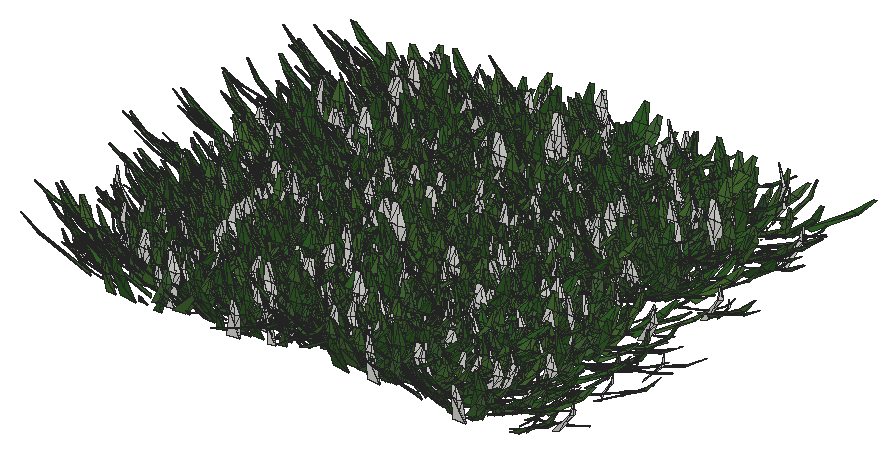
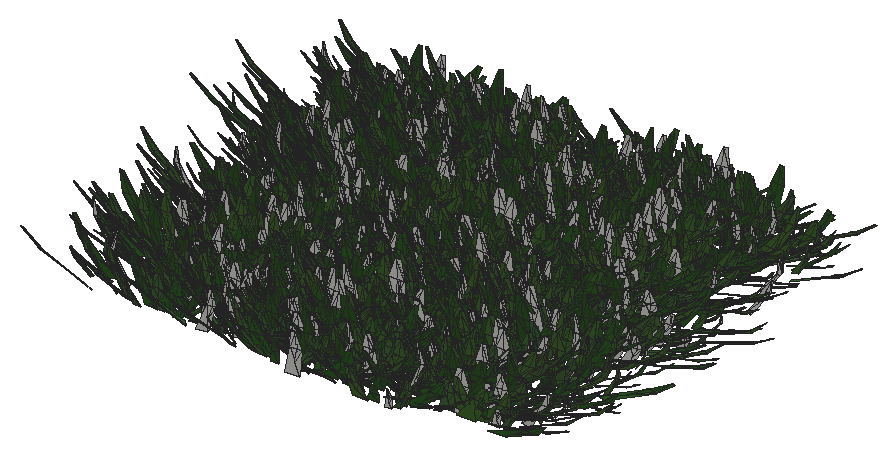
# SketchUp Ruby script. Lengths in inches.
U = 1.inch
M = Sketchup.active_model
def pt(a) = Geom::Point3d.new(a.map { |v| v * U })
def face(e, loops, mat)
  f = e.add_face(loops[0].map { |a| pt(a) })
  loops[1..].each { |l| e.add_face(l.map { |a| pt(a) }).erase! }
  f.material = f.back_material = mat if mat
  f
end
# faces: each face lists its corners as indices into pts; further lists are holes
def faces(e, pts, list, mat = nil) = list.each { |f| face(e, (f[0].is_a?(Array) ? f : [f]).map { |l| l.map { |i| pts[i] } }, mat) }
# xy, xz, yz: faces in a plane at the given z, y or x. An outline is a flat list of corners, or four numbers for a rectangle; further outlines are holes
def ring(l) = l.size == 4 ? [[l[0], l[1]], [l[2], l[1]], [l[2], l[3]], [l[0], l[3]]] : l.each_slice(2).to_a
def flat(e, list, mat, &to3) = list.each { |f| face(e, (f[0].is_a?(Array) ? f : [f]).map { |l| ring(l).map { |u, v| to3.(u, v) } }, mat) }
def xy(e, z, list, mat = nil) = flat(e, list, mat) { |x, y| [x, y, z] }
def xz(e, y, list, mat = nil) = flat(e, list, mat) { |x, z| [x, y, z] }
def yz(e, x, list, mat = nil) = flat(e, list, mat) { |y, z| [x, y, z] }
def lines(e, pts, list) = list.each { |a, b| e.add_line(pt(pts[a]), pt(pts[b])) }
# prism: a flat outline (further loops are holes) pulled along v
def prism(e, loops, v, mat = nil)
  f = face(e, loops, mat); d = Geom::Vector3d.new(v.map { |x| x * U })
  f.pushpull(f.normal.samedirection?(d) ? d.length : -d.length)
end
def box(e, o, s, mat = nil) = prism(e, [[o, [o[0] + s[0], o[1], o[2]], [o[0] + s[0], o[1] + s[1], o[2]], [o[0], o[1] + s[1], o[2]]]], [0, 0, s[2]], mat)
def at(x, y, z, deg = 0) = Geom::Transformation.translation(pt([x, y, z])) * Geom::Transformation.rotation(ORIGIN, Z_AXIS, deg.degrees)
def axes(o, x, y, z) = Geom::Transformation.new([*x, 0, *y, 0, *z, 0, *pt(o).to_a, 1])
def part(name) = M.definitions.add(name)
# library, detail: a bought-in or finely detailed component or shape, given as its bounding box
def library(name, o, s) = part(name).tap { |d| box(d.entities, o, s) }
def detail(e, o, s) = box(e.add_group.entities, o, s)
def put(e, d, t, mat = nil) = e.add_instance(d, t).tap { |i| i.material = mat if mat }
def group(e, t, mat = nil) = e.add_group.tap { |g| g.transformation = t; g.material = mat if mat }.entities
root = M.entities
M.materials.add("Material10").color = [48, 100, 38]
M.materials.add("Material3").color = [68, 110, 58]
M.materials.add("Material4").color = [48, 90, 38]
M.materials.add("Material5").color = [68, 110, 48]
M.materials.add("Material6").color = [48, 90, 48]
M.materials.add("Material7").color = [58, 110, 58]
M.materials.add("Material8").color = [58, 90, 38]
M.materials.add("Material9").color = [68, 100, 58]
c1 = part("grass00")
p = [[-0.6875,0.15,0],[-0.56,0.08,5.52],[-0.04,0.03,2.76],[0.48,-0.02,0],[0.35,-0.02,5.52],[-0.1,-0.14,5.52],
  [-0.12,0.65,8.37],[-0.42,0.65,8.37]]
faces(c1.entities,p,[[0,1,2,3],[3,2,4],[1,5,2],[5,4,2],[1,6,5],[4,5,6],[7,6,1]])
c2 = part("Group16\#1")
put(c2.entities,c1,axes([1.44,-0.61,-0.01],[0.05352,0.12609,0],[-0.10704,0.04543,0.07239],[0.06664,-0.02828,0.11628]),"Material6")
put(c2.entities,c1,axes([0.76,-0.15,-0.01],[0.04676,0.24062,0],[-0.23162,0.04501,0.06642],[0.0652,-0.01267,0.23595]),"Material3")
put(c2.entities,c1,axes([0.79,0.01,-0.01],[-0.00606,0.34651,0],[-0.34381,-0.00602,0.0432],[0.04319,0.00076,0.34386]))
put(c2.entities,c1,axes([1,0.23,-0.01],[-0.07192,0.31144,0],[-0.28722,-0.06632,0.1236],[0.12043,0.02781,0.29478]),"Material5")
put(c2.entities,c1,axes([1.66,0.77,-0.01],[-0.13828,0.29651,0],[-0.21551,-0.1005,0.22471],[0.20365,0.09498,0.23779]),"Material10")
put(c2.entities,c1,axes([0.6875,0.52,-0.01],[-0.18126,0.24051,0],[-0.22746,-0.17142,0.09788],[0.07817,0.05891,0.28481]),"Material5")
put(c2.entities,c1,axes([0.68,0.78,-0.01],[-0.215,0.18688,0],[-0.12385,-0.14248,0.21334],[0.13995,0.16101,0.18878]),"Material3")
put(c2.entities,c1,axes([0.56,1,-0.01],[-0.13756,0.07624,0],[-0.06159,-0.11112,0.0927],[0.04494,0.08108,0.12705]),"Material5")
put(c2.entities,c1,axes([0.2,0.64,-0.01],[-0.23729,0.07254,0],[-0.05711,-0.18681,0.153],[0.04473,0.14632,0.19535]),"Material10")
put(c2.entities,c1,axes([0.0625,0.72,-0.01],[-0.28874,0.02525,0],[-0.02179,-0.24916,0.14647],[0.01276,0.14591,0.25012]),"Material3")
put(c2.entities,c1,axes([-0.08,0.62,-0.01],[-0.34089,-0.04187,0],[0.03255,-0.26504,0.216],[-0.02633,0.21439,0.26703]),"Material10")
put(c2.entities,c1,axes([-0.34,0.98,-0.01],[-0.14314,-0.0493,0],[0.04397,-0.12769,0.06843],[-0.02228,0.0647,0.13505]),"Material10")
put(c2.entities,c1,axes([-0.87,1.45,-0.01],[-0.23488,-0.14114,0],[0.13761,-0.22901,0.06087],[-0.03135,0.05217,0.26717]))
put(c2.entities,c1,axes([-0.72,0.77,-0.01],[-0.14208,-0.13251,0],[0.07209,-0.0773,0.16301],[-0.11118,0.11922,0.1057]),"Material10")
put(c2.entities,c1,axes([-0.62,0.43,-0.01],[-0.14845,-0.21203,0],[0.18654,-0.13061,0.12304],[-0.10079,0.07057,0.22772]),"Material3")
put(c2.entities,c1,axes([-0.68,0.29,-0.01],[-0.13639,-0.32136,0],[0.31723,-0.13464,0.05579],[-0.05136,0.0218,0.34462]),"Material4")
put(c2.entities,c1,axes([-0.64,0.125,-0.01],[-0.0458,-0.23569,0],[0.22124,-0.043,0.08276],[-0.08124,0.01579,0.22538]),"Material7")
put(c2.entities,c1,axes([-1.6,-0.03,-0.01],[0.00576,-0.32897,0],[0.27526,0.00482,0.18018],[-0.18015,-0.00315,0.2753]),"Material5")
put(c2.entities,c1,axes([-1.36,-0.31,-0.01],[0.05718,-0.24765,0],[0.18172,0.04196,0.17267],[-0.16825,-0.03885,0.1865]),"Material10")
put(c2.entities,c1,axes([-1.54,-0.72,-0.01],[0.06537,-0.14017,0],[0.13555,0.06321,0.03939],[-0.0357,-0.01665,0.14956]))
put(c2.entities,c1,axes([-1.19,-0.9,-0.01],[0.09597,-0.12735,0],[0.11214,0.08451,0.07557],[-0.06035,-0.04548,0.14042]),"Material9")
put(c2.entities,c1,axes([-0.47,-0.54,-0.01],[0.11588,-0.10072,0],[0.0618,0.0711,0.12124],[-0.07953,-0.0915,0.0942]))
put(c2.entities,c1,axes([-0.47,-0.84,-0.01],[0.11927,-0.0661,0],[0.06603,0.11913,0.00646],[-0.00313,-0.00565,0.13621]),"Material5")
put(c2.entities,c1,axes([-0.38,-1.24,-0.01],[0.28037,-0.08571,0],[0.0618,0.20215,0.20315],[-0.05939,-0.19428,0.21139]),"Material9")
put(c2.entities,c1,axes([-0.06,-0.66,-0.01],[0.22719,-0.01987,0],[0.01247,0.14255,0.17758],[-0.01547,-0.17691,0.1431]),"Material8")
put(c2.entities,c1,axes([0.11,-0.89,-0.01],[0.14882,0.01828,0],[-0.01058,0.08611,0.12229],[0.01491,-0.12138,0.08676]),"Material6")
put(c2.entities,c1,axes([0.25,-0.72,-0.01],[0.20481,0.07053,0],[-0.06206,0.18022,0.10291],[0.03351,-0.0973,0.1906]),"Material6")
put(c2.entities,c1,axes([0.85,-1.42,-0.01],[0.16481,0.09904,0],[-0.09472,0.15762,0.05616],[0.02893,-0.04814,0.18389]),"Material5")
put(c2.entities,c1,axes([1.01,-1.09,-0.01],[0.21858,0.20385,0],[-0.17495,0.1876,0.15339],[0.10462,-0.11218,0.25652]),"Material10")
put(c2.entities,c1,axes([1.01,-0.71,-0.01],[0.08733,0.12473,0],[-0.06445,0.04512,0.13037],[0.1068,-0.07477,0.07867]),"Material6")
c3 = part("Group15\#1")
put(c3.entities,c2,at(0,0,0))
c4 = part("3darcstudiotree_grass00\#1")
put(c4.entities,c3,at(0,0,0))
put(root,c4,axes([1027.47,924.77,0],[-4.47721,-0.33604,0],[1.36403,-1.13585,-0.01736],[0.02251,-0.01875,1.33702]))
put(root,c4,axes([1027.28,911.91,0],[1.8365,-1.07849,0],[4.69569,0.49975,-0.03539],[0.15489,0.01648,1.51703]))
put(root,c4,axes([1027.77,922.46,0],[-2.97525,-0.81655,0],[2.97657,-0.67786,-0.02128],[0.12207,-0.0278,1.95268]))
put(root,c4,axes([1028.04,897.93,0],[-3.29866,-0.81098,0],[2.55083,-0.64847,-0.00764],[0.04274,-0.01087,1.81511]))
put(root,c4,axes([1028.09,930.41,0],[0.28036,-1.11473,0],[4.12363,0.06482,-0.00515],[0.03488,0.00055,1.75106]))
put(root,c4,axes([1027,915.5,0],[-2.06266,0.86143,0],[-3.87268,-0.57956,-0.03562],[-0.14938,-0.02236,1.37892]))
put(root,c4,axes([1027.79,895.99,0],[0.38604,-0.97045,0],[3.84574,0.09561,-0.03727],[0.26595,0.00661,1.73202]))
put(root,c4,axes([1028.09,899.97,0],[-3.76521,0.1423,0],[-0.75972,-1.25635,-0.03474],[-0.02334,-0.0386,1.42794]))
put(root,c4,axes([1027.06,906.23,0],[-0.0845,1.11929,0],[-4.4686,-0.02108,-0.05443],[-0.30573,-0.00144,1.56933]))
put(root,c4,axes([1028.75,921.18,0],[1.4049,-0.85059,0],[4.43609,0.45793,-0.04448],[0.26457,0.02731,1.93016]))
put(root,c4,axes([1029.04,927.01,0],[-0.32645,-1.07416,0],[4.58767,-0.08714,-0.05563],[0.36288,-0.00689,1.88098]))
put(root,c4,axes([1028.87,919.27,0],[-0.59232,1.12492,0],[-3.6265,-0.11934,-0.03263],[-0.21174,-0.00697,1.49628]))
put(root,c4,axes([1029.08,918.2,0],[4.0581,-0.29722,0],[1.26127,1.0763,-0.01036],[0.0201,0.01715,1.93559]))
put(root,c4,axes([1029.625,894.12,0],[3.20529,-0.95815,0],[3.41522,0.71406,-0.02296],[0.11616,0.02429,1.8355]))
put(root,c4,axes([1029.4,931.6,0],[-1.06603,0.92748,0],[-4.93521,-0.35453,-0.06106],[-0.26936,-0.01935,1.47293]))
put(root,c4,axes([1029.21,910.23,0],[5.08676,-0.19422,0],[0.58185,0.95246,-0.02943],[0.02798,0.0458,1.51666]))
put(root,c4,axes([1030.8,908.57,0],[-0.19939,-1.04542,0],[4.4829,-0.05344,-0.05646],[0.31576,-0.00376,1.57058]))
put(root,c4,axes([1029.35,901.36,0],[2.71383,0.81638,0],[-3.43896,0.71449,-0.05468],[-0.2392,0.0497,1.58958]))
put(root,c4,axes([1029.31,916.84,0],[4.84098,0.43489,0],[-1.61189,1.12141,-0.03831],[-0.06664,0.04636,1.53223]))
put(root,c4,axes([1029.89,928.53,0],[4.94595,-0.11829,0],[0.37031,0.96768,-0.00501],[0.00319,0.00833,1.62495]))
put(root,c4,axes([1029.56,902.87,0],[2.55592,1.10469,0],[-4.04438,0.58485,-0.02506],[-0.13578,0.01964,1.82822]))
put(root,c4,axes([1030.2,897.16,0],[4.08301,-0.07651,0],[0.38191,1.27383,-0.00347],[0.00157,0.00523,1.92949]))
put(root,c4,axes([1031.29,925.83,0],[-2.35704,0.79519,0],[-3.72282,-0.68968,-0.05517],[-0.2648,-0.04906,1.72999]))
put(root,c4,axes([1030.53,907.58,0],[2.61917,0.95948,0],[-3.03892,0.51848,-0.01403],[-0.09978,0.01702,1.97952]))
put(root,c4,axes([1030.63,913.6,0],[3.34714,0.66833,0],[-2.79001,0.87331,-0.04015],[-0.12528,0.03922,1.39698]))
put(root,c4,axes([1031.24,904.6,0],[0.48467,1.00987,0],[-3.72895,0.11185,-0.01784],[-0.13598,0.00408,1.80168]))
put(root,c4,axes([1033.03,923.72,0],[-1.59666,-0.99905,0],[3.40836,-0.34045,-0.01431],[0.10062,-0.01005,1.73701]))
put(root,c4,axes([1033.2,895.67,0],[-3.03643,0.87412,0],[-2.8621,-0.62138,-0.01448],[-0.06458,-0.01402,1.39954]))
put(root,c4,axes([1034.26,896.73,0],[-4.02149,-0.43578,0],[1.45299,-0.83803,-0.04544],[0.11799,-0.06805,1.4908]))
put(root,c4,axes([1034.54,919.36,0],[-4.89707,0.28407,0],[-0.88262,-0.95096,-0.03599],[-0.04789,-0.0516,1.43677]))
put(root,c4,axes([1033.86,904.3,0],[-3.37258,0.90608,0],[-3.64602,-0.8482,-0.01383],[-0.04832,-0.01124,1.48532]))
put(root,c4,axes([1033.36,912.23,0],[4.28972,0.40809,0],[-1.53876,1.01093,-0.01203],[-0.02546,0.01673,1.60927]))
put(root,c4,axes([1035.4,908.85,0],[-1.14965,-0.87516,0],[3.85465,-0.31648,-0.02104],[0.11481,-0.00943,1.45661]))
put(root,c4,axes([1034.59,906.46,0],[3.45148,-0.64536,0],[2.96079,0.98967,-0.02614],[0.07518,0.02513,1.48366]))
put(root,c4,axes([1035.44,910.79,0],[-4.9983,0.12378,0],[-0.36429,-0.91937,-0.0174],[-0.01281,-0.03234,1.72585]))
put(root,c4,axes([1035.97,928.63,0],[-3.38152,-0.37053,0],[1.95757,-1.11657,-0.00176],[0.00453,-0.00258,1.95594]))
put(root,c4,axes([1034.94,901.15,0],[-2.34957,0.94392,0],[-4.17021,-0.64877,-0.04897],[-0.26523,-0.04126,1.9584]))
put(root,c4,axes([1034.35,898.87,0],[3.32402,0.3596,0],[-1.44399,0.83424,-0.02703],[-0.09074,0.05242,1.9211]))
put(root,c4,axes([1036.37,916.36,0],[-3.05623,-0.47682,0],[2.41216,-0.96631,-0.00523],[0.01811,-0.00725,1.86317]))
put(root,c4,axes([1036.51,918.73,0],[-3.75382,-0.50938,0],[2.09214,-0.9636,-0.04387],[0.13012,-0.05993,1.70431]))
put(root,c4,axes([1035.75,899.8,0],[-3.73599,0.53776,0],[-2.5701,-1.11595,-0.0199],[-0.05158,-0.02239,1.67187]))
put(root,c4,axes([1034.67,915.52,0],[1.67846,0.81167,0],[-4.27264,0.55222,-0.03477],[-0.1745,0.02255,1.69826]))
put(root,c4,axes([1036.07,907.16,0],[-3.09646,0.77516,0],[-3.18498,-0.79517,-0.05526],[-0.23608,-0.05894,1.69871]))
put(root,c4,axes([1036.09,902.59,0],[2.62671,-0.96021,0],[3.1714,0.54222,-0.02882],[0.14083,0.02408,1.42183]))
put(root,c4,axes([1036.55,933.42,0],[0.41254,-1.11538,0],[3.92373,0.0907,-0.04487],[0.25663,0.00593,1.41449]))
put(root,c4,axes([1037,932.375,0],[-4.83141,-0.06367,0],[0.25709,-1.21932,-0.0488],[0.01394,-0.06614,1.65721]))
put(root,c4,axes([1036.85,894.42,0],[-3.80323,0.13534,0],[-0.55678,-0.97788,-0.03826],[-0.03613,-0.06345,1.65468]))
put(root,c4,axes([1037.46,929.85,0],[-4.67907,-0.20575,0],[0.86048,-1.22305,-0.04722],[0.03699,-0.05257,1.40384]))
put(root,c4,axes([1035.99,926.74,0],[-1.05875,1.15742,0],[-4.29725,-0.24568,-0.0233],[-0.13048,-0.00746,1.58282]))
put(root,c4,axes([1036.05,913.77,0],[4.14871,0.66652,0],[-2.80307,1.09047,-0.03131],[-0.07779,0.03026,1.48921]))
put(root,c4,axes([1036.3125,922.79,0],[2.97201,1.00736,0],[-3.97981,0.73385,-0.05484],[-0.18767,0.03461,1.31443]))
put(root,c4,axes([1036.93,921.4,0],[3.73635,0.02915,0],[-0.121,0.9694,-0.01718],[-0.00416,0.0333,1.88076]))
put(root,c4,axes([1039.2,906.45,0],[-3.38708,-0.63927,0],[2.81669,-0.93274,-0.01411],[0.04933,-0.01634,1.69584]))
put(root,c4,axes([1037.17,925.41,0],[0.16986,1.07544,0],[-5.18803,0.05121,-0.04149],[-0.19714,0.00195,1.54325]))
put(root,c4,axes([1039.4,919.5,0],[0.73918,-1.25402,0],[4.5803,0.16874,-0.00777],[0.03593,0.00132,1.3523]))
put(root,c4,axes([1039.57,916.7,0],[-0.83171,-0.90909,0],[4.59832,-0.26293,-0.04627],[0.28513,-0.0163,1.86363]))
put(root,c4,axes([1039.62,907.2,0],[-4.52783,0.09424,0],[-0.31079,-0.93327,-0.02559],[-0.01771,-0.05318,1.95328]))
put(root,c4,axes([1040.47,915.05,0],[1.09611,-0.92163,0],[4.84666,0.36027,-0.06029],[0.32691,0.0243,1.78762]))
put(root,c4,axes([1040.14,929.75,0],[2.30561,-0.85947,0],[4.07199,0.68272,-0.05795],[0.30529,0.05118,1.94389]))
put(root,c4,axes([1039.42,898.43,0],[4.15645,0.11327,0],[-0.40548,0.92998,-0.03498],[-0.02406,0.05518,1.48455]))
put(root,c4,axes([1040.35,911.98,0],[-3.28835,0.69112,0],[-2.3207,-0.69011,-0.00081],[-0.00409,-0.00122,1.76997]))
put(root,c4,axes([1041.58,924.61,0],[-0.05217,-0.99103,0],[4.9332,-0.01623,-0.00745],[0.04692,-0.00015,1.94284]))
put(root,c4,axes([1040.15,895.47,0],[0.29849,1.1081,0],[-3.91006,0.06583,-0.04154],[-0.31526,0.00531,1.86323]))
put(root,c4,axes([1041.73,921.3,0],[-4.94093,-0.24625,0],[0.95755,-1.20083,-0.01918],[0.02332,-0.02924,1.90358]))
put(root,c4,axes([1040.38,926.125,0],[3.27459,-0.53526,0],[2.01,0.76855,-0.045],[0.14728,0.05631,1.37282]))
put(root,c4,axes([1041.78,910.82,0],[0.57888,-1.02767,0],[4.86352,0.17122,-0.00524],[0.03332,0.00117,1.97007]))
put(root,c4,axes([1039.92,903.49,0],[1.77436,0.79751,0],[-3.18659,0.44311,-0.00131],[-0.00977,0.00136,1.9458]))
put(root,c4,axes([1041.04,896.86,0],[-3.36301,0.64766,0],[-2.44825,-0.79454,-0.00087],[-0.00355,-0.00115,1.68429]))
put(root,c4,axes([1042.18,901.27,0],[-1.4545,-0.88118,0],[4.51048,-0.46532,-0.01762],[0.07914,-0.00816,1.48208]))
put(root,c4,axes([1040.09,899.62,0],[3.81768,0.66428,0],[-2.44879,0.87959,-0.01513],[-0.0462,0.0166,1.43215]))
put(root,c4,axes([1041.28,922.59,0],[4.08726,-0.46656,0],[1.95644,1.0712,-0.05401],[0.10986,0.06015,1.44188]))
put(root,c4,axes([1043.09,931.68,0],[-3.9964,-0.52288,0],[2.12612,-1.01563,-0.05348],[0.15903,-0.07597,1.83786]))
put(root,c4,axes([1041.66,913.75,0],[4.81145,-0.0979,0],[0.38638,1.1868,-0.02372],[0.00959,0.02946,1.48337]))
put(root,c4,axes([1043.29,932.78,0],[-4.62401,0.29061,0],[-0.94259,-0.93738,-0.03206],[-0.05298,-0.05269,1.63785]))
put(root,c4,axes([1042.22,927.08,0],[2.68838,0.69195,0],[-3.43987,0.83529,-0.03466],[-0.15751,0.03825,1.89896]))
put(root,c4,axes([1042.27,917.97,0],[3.81617,0.61886,0],[-2.68846,1.03615,-0.05832],[-0.15316,0.05903,1.48992]))
put(root,c4,axes([1042.85,928.94,0],[-0.04272,0.99569,0],[-4.10213,-0.011,-0.03184],[-0.21296,-0.00057,1.71482]))
put(root,c4,axes([1043.27,909.27,0],[-2.13592,1.02189,0],[-4.55643,-0.59523,-0.06253],[-0.32722,-0.04275,1.89715]))
put(root,c4,axes([1043.16,904.68,0],[3.87992,-0.06992,0],[0.26674,0.92505,-0.00836],[0.00512,0.01775,1.97523]))
put(root,c4,axes([1045.57,916.74,0],[-3.92726,-0.53289,0],[2.331,-1.07368,-0.04044],[0.11775,-0.05424,1.86421]))
put(root,c4,axes([1045.87,913.58,0],[-4.06696,-0.33259,0],[1.16201,-0.88807,-0.035],[0.08068,-0.06166,1.73222]))
put(root,c4,axes([1046.48,927.5625,0],[-4.12513,-0.57559,0],[2.48785,-1.11437,-0.0179],[0.04452,-0.01994,1.62858]))
put(root,c4,axes([1045.56,901.41,0],[-3.59802,0.5872,0],[-2.6694,-1.02229,-0.04574],[-0.15156,-0.05804,1.85022]))
put(root,c4,axes([1046.375,900.48,0],[0.47235,-1.15777,0],[4.32597,0.11031,-0.00761],[0.05408,0.00138,1.94156]))
put(root,c4,axes([1046.66,919.28,0],[-3.32765,-0.85792,0],[3.0305,-0.73466,-0.04714],[0.2036,-0.04936,1.58733]))
put(root,c4,axes([1045.11,897.97,0],[5.16492,-0.13655,0],[0.53557,1.26611,-0.02611],[0.01692,0.04001,1.96192]))
put(root,c4,axes([1046.31,921.05,0],[-3.3634,0.85391,0],[-3.17768,-0.78227,-0.02428],[-0.08249,-0.02031,1.32917]))
put(root,c4,axes([1047.3,903.51,0],[-3.44,-0.36745,0],[1.97613,-1.15625,-0.04539],[0.10919,-0.06389,1.92461]))
put(root,c4,axes([1045.9,933.73,0],[4.78852,-0.11236,0],[0.42706,1.13749,-0.03728],[0.02321,0.06182,1.90298]))
put(root,c4,axes([1046.29,929.87,0],[4.63211,-0.48455,0],[1.59506,0.95302,-0.04818],[0.10631,0.06352,1.47658]))
put(root,c4,axes([1046.57,929.2,0],[3.86267,-0.07613,0],[0.40494,1.28409,-0.03935],[0.01388,0.04402,1.44542]))
put(root,c4,axes([1047.37,923.84,0],[2.43686,-0.68298,0],[3.57771,0.79783,-0.04874],[0.17486,0.03899,1.44038]))
put(root,c4,axes([1046.5,906.1,0],[4.82681,-0.00126,0],[0.00513,1.22505,-0.04894],[0.00024,0.05639,1.41164]))
put(root,c4,axes([1048.57,918.72,0],[-3.42276,-0.65167,0],[2.58269,-0.84782,-0.01582],[0.04944,-0.01623,1.37394]))
put(root,c4,axes([1047.43,915.64,0],[-2.36541,1.04526,0],[-3.84689,-0.54409,-0.02589],[-0.11432,-0.01617,1.40149]))
put(root,c4,axes([1047.96,931.86,0],[2.7424,-0.7825,0],[2.89337,0.63377,-0.00209],[0.01007,0.00221,1.54397]))
put(root,c4,axes([1048.125,926.05,0],[-4.1603,0.72793,0],[-2.33598,-0.83442,-0.01309],[-0.05536,-0.01977,1.87779]))
put(root,c4,axes([1048.86,905.07,0],[-0.84808,-1.10481,0],[3.74786,-0.17981,-0.00431],[0.02392,-0.00115,1.34772]))
put(root,c4,axes([1049.17,895.875,0],[-1.71072,-0.80836,0],[3.80701,-0.50355,-0.0302],[0.16613,-0.02197,1.67548]))
put(root,c4,axes([1049.26,908.88,0],[0.18531,-0.97415,0],[3.90679,0.04645,-0.0123],[0.08869,0.00105,1.7643]))
put(root,c4,axes([1047.97,911.875,0],[3.52409,0.23962,0],[-1.16841,1.07399,-0.02379],[-0.03363,0.03091,1.49895]))
put(root,c4,axes([1047.71,907.51,0],[1.29524,0.85298,0],[-4.77119,0.45281,-0.02635],[-0.13125,0.01246,1.69955]))
put(root,c4,axes([1049.53,922.7,0],[-4.98991,0.20865,0],[-0.7989,-1.19409,-0.00717],[-0.00589,-0.0088,1.50735]))
put(root,c4,axes([1048.97,910.96,0],[2.92176,-0.52894,0],[2.46205,0.84999,-0.04376],[0.17079,0.05896,1.7457]))
put(root,c4,axes([1051.27,916.21,0],[-2.67053,-0.99485,0],[3.36476,-0.56452,-0.00883],[0.05512,-0.00925,1.90461]))
put(root,c4,axes([1051.68,929,0],[-2.95255,-0.81537,0],[3.60487,-0.81585,-0.01753],[0.06331,-0.01433,1.48083]))
put(root,c4,axes([1049.44,896.98,0],[-0.18508,1.23432,0],[-4.73712,-0.04439,-0.00219],[-0.0103,-0.0001,1.39308]))
put(root,c4,axes([1051.89,899.52,0],[-4.20317,-0.73758,0],[2.25744,-0.80401,-0.02484],[0.09654,-0.03438,1.66133]))
put(root,c4,axes([1051.55,924.73,0],[-4.46812,0.07741,0],[-0.25002,-0.9019,-0.01842],[-0.00759,-0.0274,1.34789]))
put(root,c4,axes([1052.08,895.75,0],[-3.42874,0.45159,0],[-1.78492,-0.84701,-0.01732],[-0.06439,-0.03056,1.90951]))
put(root,c4,axes([1053.4,932.08,0],[-1.47134,-1.07173,0],[4.62951,-0.39723,-0.00214],[0.01137,-0.00098,1.72072]))
put(root,c4,axes([1051.28,900.98,0],[4.20048,0.55778,0],[-1.88075,0.88521,-0.04207],[-0.14917,0.07021,1.89419]))
put(root,c4,axes([1051.74,912.16,0],[2.35176,0.86373,0],[-3.11236,0.52965,-0.02533],[-0.14132,0.02405,1.58831]))
put(root,c4,axes([1052.4,927.66,0],[4.3887,-0.53019,0],[1.93978,1.00355,-0.00312],[0.00847,0.00438,1.73901]))
put(root,c4,axes([1052.07,907.65,0],[1.01063,1.23996,0],[-4.41491,0.2249,-0.0503],[-0.27557,0.01404,1.57458]))
put(root,c4,axes([1052.4375,918.11,0],[-1.65132,1.02753,0],[-4.1479,-0.41662,-0.02547],[-0.11726,-0.01178,1.38631]))
put(root,c4,axes([1053.59,905.59,0],[0.96836,-1.19447,0],[4.79826,0.24312,-0.041],[0.23189,0.01175,1.76588]))
put(root,c4,axes([1052.3,902.74,0],[4.53801,0.33747,0],[-1.32832,1.11639,-0.03162],[-0.04162,0.03498,1.3441]))
put(root,c4,axes([1052.14,913.24,0],[2.33175,0.74132,0],[-3.89169,0.76506,-0.01217],[-0.05632,0.01107,1.82194]))
put(root,c4,axes([1053.86,896.51,0],[1.73115,-0.99463,0],[4.00302,0.43545,-0.04597],[0.21468,0.02335,1.38947]))
put(root,c4,axes([1054.84,898.8125,0],[-4.68105,-0.44507,0],[1.39415,-0.91644,-0.04106],[0.1024,-0.06731,1.71966]))
put(root,c4,axes([1054.75,929.99,0],[-4.10991,0.05659,0],[-0.25803,-1.17127,-0.02509],[-0.00633,-0.02875,1.34616]))
put(root,c4,axes([1055.46,923.29,0],[-0.81845,-1.22057,0],[4.38476,-0.18376,-0.02808],[0.16711,-0.007,1.67665]))
put(root,c4,axes([1054.63,910.26,0],[2.60124,-1.09423,0],[3.31981,0.49325,-0.0411],[0.22316,0.03316,1.52451]))
put(root,c4,axes([1053.76,919.62,0],[3.5289,0.32153,0],[-1.76569,1.21119,-0.03532],[-0.06738,0.04622,1.79519]))
put(root,c4,axes([1054.29,915.71,0],[0.58187,0.98724,0],[-3.75225,0.13822,-0.04131],[-0.23221,0.00855,1.34689]))
put(root,c4,axes([1054.82,909.6,0],[4.31659,-0.72181,0],[2.02591,0.75722,-0.03191],[0.13976,0.05224,1.79443]))
put(root,c4,axes([1055.25,904.55,0],[3.90895,-0.31621,0],[1.44431,1.11591,-0.01717],[0.02682,0.02072,1.48777]))
put(root,c4,axes([1055.33,920.79,0],[0.60806,1.1895,0],[-3.81317,0.12183,-0.04145],[-0.33743,0.01078,1.97198]))
put(root,c4,axes([1055.06,925.64,0],[4.01339,0.62208,0],[-2.19682,0.88582,-0.03504],[-0.13521,0.05452,1.90819]))
put(root,c4,axes([1057.48,899.92,0],[-1.20844,-0.99932,0],[4.83991,-0.36579,-0.03772],[0.15637,-0.01182,1.36861]))
put(root,c4,axes([1057.26,920.68,0],[-2.41677,0.79192,0],[-3.38406,-0.64546,-0.05103],[-0.26235,-0.05004,1.72023]))
put(root,c4,axes([1057.77,929.03,0],[-3.63977,0.77847,0],[-2.95769,-0.8643,-0.05065],[-0.16741,-0.04892,1.44592]))
put(root,c4,axes([1058.95,918.44,0],[-3.02666,-0.90444,0],[3.4297,-0.71733,-0.01878],[0.08665,-0.01812,1.68146]))
put(root,c4,axes([1059.2,913.39,0],[-3.4696,-0.46787,0],[1.78358,-0.82666,-0.04409],[0.13229,-0.06131,1.48398]))
put(root,c4,axes([1058.9375,919.18,0],[-4.56638,0.55078,0],[-1.82444,-0.94538,-0.02532],[-0.06885,-0.03568,1.64221]))
put(root,c4,axes([1057.8,933.28,0],[4.17819,0.33382,0],[-1.2451,0.97401,-0.03842],[-0.08739,0.06836,1.90991]))
put(root,c4,axes([1058.47,908.57,0],[4.13559,-0.54308,0],[1.81906,0.86577,-0.02304],[0.07821,0.03723,1.78453]))
put(root,c4,axes([1060.14,927.46,0],[0.6928,-1.22893,0],[4.48898,0.15816,-0.02402],[0.15455,0.00545,1.84088]))
put(root,c4,axes([1060.3,902.66,0],[-4.87146,0.02178,0],[-0.08116,-1.13448,-0.01042],[-0.0012,-0.01672,1.82123]))
put(root,c4,axes([1060.28,895.11,0],[-3.73268,0.3096,0],[-1.29853,-0.97848,-0.04681],[-0.08807,-0.06636,1.53984]))
put(root,c4,axes([1058.92,901.8,0],[3.88196,0.27706,0],[-1.31813,1.15428,-0.00872],[-0.01209,0.01059,1.51538]))
put(root,c4,axes([1059.61,922.625,0],[-0.31756,1.20415,0],[-3.66526,-0.06041,-0.03816],[-0.32346,-0.00533,1.95014]))
put(root,c4,axes([1058.75,898.19,0],[3.73866,0.84444,0],[-2.52225,0.69793,-0.00582],[-0.02595,0.00718,1.56404]))
put(root,c4,axes([1058.89,906.13,0],[3.21656,0.87415,0],[-3.40413,0.78287,-0.033],[-0.15769,0.03627,1.87715]))
put(root,c4,axes([1061.26,907.22,0],[-1.25696,-0.97634,0],[4.48228,-0.36066,-0.0477],[0.21367,-0.01719,1.385]))
put(root,c4,axes([1061.68,897.4,0],[-2.73694,-0.75436,0],[3.09304,-0.70138,-0.0539],[0.21901,-0.04966,1.43163]))
put(root,c4,axes([1059.92,910.96,0],[3.21354,0.61237,0],[-2.33536,0.76595,-0.01463],[-0.06404,0.021,1.73802]))
